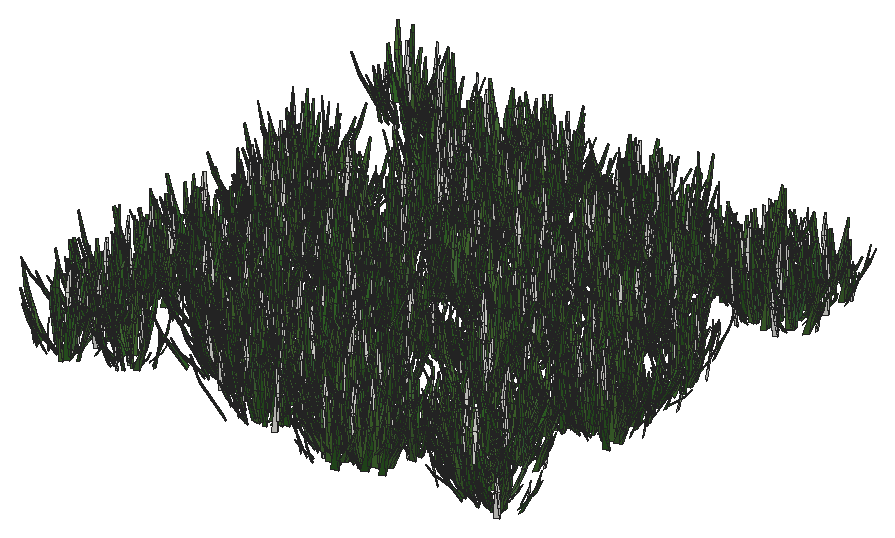
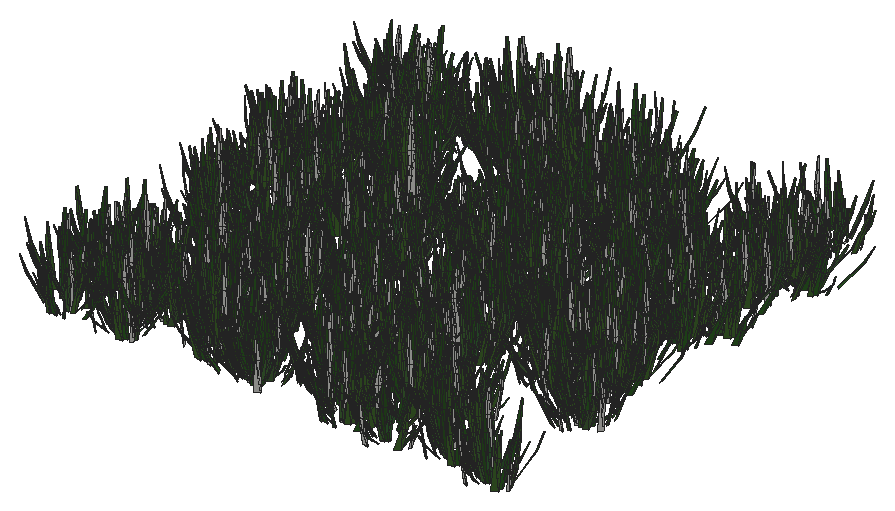
# SketchUp Ruby script. Lengths in inches.
U = 1.inch
M = Sketchup.active_model
def pt(a) = Geom::Point3d.new(a.map { |v| v * U })
def face(e, loops, mat)
  f = e.add_face(loops[0].map { |a| pt(a) })
  loops[1..].each { |l| e.add_face(l.map { |a| pt(a) }).erase! }
  f.material = f.back_material = mat if mat
  f
end
# faces: each face lists its corners as indices into pts; further lists are holes
def faces(e, pts, list, mat = nil) = list.each { |f| face(e, (f[0].is_a?(Array) ? f : [f]).map { |l| l.map { |i| pts[i] } }, mat) }
# xy, xz, yz: faces in a plane at the given z, y or x. An outline is a flat list of corners, or four numbers for a rectangle; further outlines are holes
def ring(l) = l.size == 4 ? [[l[0], l[1]], [l[2], l[1]], [l[2], l[3]], [l[0], l[3]]] : l.each_slice(2).to_a
def flat(e, list, mat, &to3) = list.each { |f| face(e, (f[0].is_a?(Array) ? f : [f]).map { |l| ring(l).map { |u, v| to3.(u, v) } }, mat) }
def xy(e, z, list, mat = nil) = flat(e, list, mat) { |x, y| [x, y, z] }
def xz(e, y, list, mat = nil) = flat(e, list, mat) { |x, z| [x, y, z] }
def yz(e, x, list, mat = nil) = flat(e, list, mat) { |y, z| [x, y, z] }
def lines(e, pts, list) = list.each { |a, b| e.add_line(pt(pts[a]), pt(pts[b])) }
# prism: a flat outline (further loops are holes) pulled along v
def prism(e, loops, v, mat = nil)
  f = face(e, loops, mat); d = Geom::Vector3d.new(v.map { |x| x * U })
  f.pushpull(f.normal.samedirection?(d) ? d.length : -d.length)
end
def box(e, o, s, mat = nil) = prism(e, [[o, [o[0] + s[0], o[1], o[2]], [o[0] + s[0], o[1] + s[1], o[2]], [o[0], o[1] + s[1], o[2]]]], [0, 0, s[2]], mat)
def at(x, y, z, deg = 0) = Geom::Transformation.translation(pt([x, y, z])) * Geom::Transformation.rotation(ORIGIN, Z_AXIS, deg.degrees)
def axes(o, x, y, z) = Geom::Transformation.new([*x, 0, *y, 0, *z, 0, *pt(o).to_a, 1])
def part(name) = M.definitions.add(name)
# library, detail: a bought-in or finely detailed component or shape, given as its bounding box
def library(name, o, s) = part(name).tap { |d| box(d.entities, o, s) }
def detail(e, o, s) = box(e.add_group.entities, o, s)
def put(e, d, t, mat = nil) = e.add_instance(d, t).tap { |i| i.material = mat if mat }
def group(e, t, mat = nil) = e.add_group.tap { |g| g.transformation = t; g.material = mat if mat }.entities
root = M.entities
M.materials.add("Material1").color = [58, 110, 58]
M.materials.add("Material10").color = [48, 100, 38]
M.materials.add("Material3").color = [68, 110, 58]
M.materials.add("Material4").color = [48, 90, 38]
M.materials.add("Material5").color = [68, 110, 48]
M.materials.add("Material6").color = [48, 90, 48]
M.materials.add("Material8").color = [58, 90, 38]
M.materials.add("Material9").color = [68, 100, 58]
c1 = part("grass00")
p = [[-0.6875,0.15,0],[-0.56,0.08,5.52],[-0.04,0.03,2.76],[0.48,-0.02,0],[0.35,-0.02,5.52],[-0.1,-0.14,5.52],
  [-0.12,0.65,8.37],[-0.42,0.65,8.37]]
faces(c1.entities,p,[[0,1,2,3],[3,2,4],[1,5,2],[5,4,2],[1,6,5],[4,5,6],[7,6,1]])
c2 = part("Group16\#1")
put(c2.entities,c1,axes([1.44,-0.61,-0.01],[0.05352,0.12609,0],[-0.10704,0.04543,0.07239],[0.06664,-0.02828,0.11628]),"Material6")
put(c2.entities,c1,axes([0.76,-0.15,-0.01],[0.04676,0.24062,0],[-0.23162,0.04501,0.06642],[0.0652,-0.01267,0.23595]),"Material3")
put(c2.entities,c1,axes([0.79,0.01,-0.01],[-0.00606,0.34651,0],[-0.34381,-0.00602,0.0432],[0.04319,0.00076,0.34386]))
put(c2.entities,c1,axes([1,0.23,-0.01],[-0.07192,0.31144,0],[-0.28722,-0.06632,0.1236],[0.12043,0.02781,0.29478]),"Material5")
put(c2.entities,c1,axes([1.66,0.77,-0.01],[-0.13828,0.29651,0],[-0.21551,-0.1005,0.22471],[0.20365,0.09498,0.23779]),"Material10")
put(c2.entities,c1,axes([0.6875,0.52,-0.01],[-0.18126,0.24051,0],[-0.22746,-0.17142,0.09788],[0.07817,0.05891,0.28481]),"Material5")
put(c2.entities,c1,axes([0.68,0.78,-0.01],[-0.215,0.18688,0],[-0.12385,-0.14248,0.21334],[0.13995,0.16101,0.18878]),"Material3")
put(c2.entities,c1,axes([0.56,1,-0.01],[-0.13756,0.07624,0],[-0.06159,-0.11112,0.0927],[0.04494,0.08108,0.12705]),"Material5")
put(c2.entities,c1,axes([0.2,0.64,-0.01],[-0.23729,0.07254,0],[-0.05711,-0.18681,0.153],[0.04473,0.14632,0.19535]),"Material10")
put(c2.entities,c1,axes([0.0625,0.72,-0.01],[-0.28874,0.02525,0],[-0.02179,-0.24916,0.14647],[0.01276,0.14591,0.25012]),"Material3")
put(c2.entities,c1,axes([-0.08,0.62,-0.01],[-0.34089,-0.04187,0],[0.03255,-0.26504,0.216],[-0.02633,0.21439,0.26703]),"Material10")
put(c2.entities,c1,axes([-0.34,0.98,-0.01],[-0.14314,-0.0493,0],[0.04397,-0.12769,0.06843],[-0.02228,0.0647,0.13505]),"Material10")
put(c2.entities,c1,axes([-0.87,1.45,-0.01],[-0.23488,-0.14114,0],[0.13761,-0.22901,0.06087],[-0.03135,0.05217,0.26717]))
put(c2.entities,c1,axes([-0.72,0.77,-0.01],[-0.14208,-0.13251,0],[0.07209,-0.0773,0.16301],[-0.11118,0.11922,0.1057]),"Material10")
put(c2.entities,c1,axes([-0.62,0.43,-0.01],[-0.14845,-0.21203,0],[0.18654,-0.13061,0.12304],[-0.10079,0.07057,0.22772]),"Material3")
put(c2.entities,c1,axes([-0.68,0.29,-0.01],[-0.13639,-0.32136,0],[0.31723,-0.13464,0.05579],[-0.05136,0.0218,0.34462]),"Material4")
put(c2.entities,c1,axes([-0.64,0.125,-0.01],[-0.0458,-0.23569,0],[0.22124,-0.043,0.08276],[-0.08124,0.01579,0.22538]),"Material1")
put(c2.entities,c1,axes([-1.6,-0.03,-0.01],[0.00576,-0.32897,0],[0.27526,0.00482,0.18018],[-0.18015,-0.00315,0.2753]),"Material5")
put(c2.entities,c1,axes([-1.36,-0.31,-0.01],[0.05718,-0.24765,0],[0.18172,0.04196,0.17267],[-0.16825,-0.03885,0.1865]),"Material10")
put(c2.entities,c1,axes([-1.54,-0.72,-0.01],[0.06537,-0.14017,0],[0.13555,0.06321,0.03939],[-0.0357,-0.01665,0.14956]))
put(c2.entities,c1,axes([-1.19,-0.9,-0.01],[0.09597,-0.12735,0],[0.11214,0.08451,0.07557],[-0.06035,-0.04548,0.14042]),"Material9")
put(c2.entities,c1,axes([-0.47,-0.54,-0.01],[0.11588,-0.10072,0],[0.0618,0.0711,0.12124],[-0.07953,-0.0915,0.0942]))
put(c2.entities,c1,axes([-0.47,-0.84,-0.01],[0.11927,-0.0661,0],[0.06603,0.11913,0.00646],[-0.00313,-0.00565,0.13621]),"Material5")
put(c2.entities,c1,axes([-0.38,-1.24,-0.01],[0.28037,-0.08571,0],[0.0618,0.20215,0.20315],[-0.05939,-0.19428,0.21139]),"Material9")
put(c2.entities,c1,axes([-0.06,-0.66,-0.01],[0.22719,-0.01987,0],[0.01247,0.14255,0.17758],[-0.01547,-0.17691,0.1431]),"Material8")
put(c2.entities,c1,axes([0.11,-0.89,-0.01],[0.14882,0.01828,0],[-0.01058,0.08611,0.12229],[0.01491,-0.12138,0.08676]),"Material6")
put(c2.entities,c1,axes([0.25,-0.72,-0.01],[0.20481,0.07053,0],[-0.06206,0.18022,0.10291],[0.03351,-0.0973,0.1906]),"Material6")
put(c2.entities,c1,axes([0.85,-1.42,-0.01],[0.16481,0.09904,0],[-0.09472,0.15762,0.05616],[0.02893,-0.04814,0.18389]),"Material5")
put(c2.entities,c1,axes([1.01,-1.09,-0.01],[0.21858,0.20385,0],[-0.17495,0.1876,0.15339],[0.10462,-0.11218,0.25652]),"Material10")
put(c2.entities,c1,axes([1.01,-0.71,-0.01],[0.08733,0.12473,0],[-0.06445,0.04512,0.13037],[0.1068,-0.07477,0.07867]),"Material6")
c3 = part("Group15\#1")
put(c3.entities,c2,at(0,0,0))
c4 = part("3darcstudiotree_grass00\#1")
put(c4.entities,c3,at(0,0,0))
put(root,c4,axes([268.16,97.04,0.25],[1.10424,-0.06793,0],[0.07798,0.87325,-0.02045],[0.00258,0.02892,1.8024]))
put(root,c4,axes([287.49,97.18,0.25],[0.30872,-0.99726,0],[1.14542,0.24428,-0.01129],[0.01726,0.00368,1.86628]))
put(root,c4,axes([288.79,97.94,0.25],[0.3848,-0.95006,0],[1.16691,0.32559,-0.02131],[0.02787,0.00778,1.69918]))
put(root,c4,axes([289.95,98.12,0.25],[0.36065,-0.88025,0],[1.08014,0.30487,-0.01889],[0.03083,0.0087,1.96679]))
put(root,c4,axes([281.65,97.91,0.25],[-1.09019,-0.50143,0],[0.60004,-0.89873,-0.02403],[0.01807,-0.02706,1.92026]))
put(root,c4,axes([271.9375,98.29,0.25],[0.34802,0.74456,0],[-0.96206,0.30978,-0.02781],[-0.03955,0.01273,1.57422]))
put(root,c4,axes([298.37,98.26,0.25],[-1.11705,-0.08782,0],[0.09396,-0.82334,-0.02721],[0.00339,-0.02975,1.31849]))
put(root,c4,axes([286.48,98.61,0.25],[0.24214,0.73963,0],[-0.93506,0.21089,-0.02204],[-0.04106,0.00926,1.87051]))
put(root,c4,axes([282.78,99.14,0.25],[1.15932,-0.25477,0],[0.28267,0.88609,-0.03329],[0.01046,0.0328,1.35616]))
put(root,c4,axes([296.02,99.06,0.25],[-0.27861,0.84951,0],[-1.24912,-0.28222,-0.0223],[-0.02643,-0.00597,1.58974]))
put(root,c4,axes([280,99.92,0.25],[0.8678,0.26913,0],[-0.39255,0.87201,-0.02415],[-0.01451,0.03224,1.92547]))
put(root,c4,axes([269.21,99.85,0.25],[-0.87323,0.18273,0],[-0.30243,-0.99566,-0.01943],[-0.00513,-0.01691,1.33771]))
put(root,c4,axes([295.06,100.45,0.25],[0.23734,-0.94344,0],[1.1996,0.20789,-0.01659],[0.02057,0.00357,1.55232]))
put(root,c4,axes([290.86,100.39,0.25],[0.77506,0.65428,0],[-0.89383,0.72943,-0.00938],[-0.01044,0.00852,1.95578]))
put(root,c4,axes([288.87,100.38,0.25],[0.63502,0.71653,0],[-0.97082,0.59271,-0.02079],[-0.01883,0.0115,1.35493]))
put(root,c4,axes([278.34,100.35,0.25],[-1.08362,-0.14985,0],[0.15604,-0.77736,-0.01531],[0.00477,-0.02379,1.80136]))
put(root,c4,axes([277.1,100.4,0.25],[-1.24003,0.01344,0],[-0.01576,-1.00201,-0.02897],[-0.00045,-0.02857,1.4344]))
put(root,c4,axes([267.86,100.45,0.25],[-1.00644,0.0521,0],[-0.07788,-1.03631,-0.0193],[-0.00128,-0.01707,1.33558]))
put(root,c4,axes([283.02,101.13,0.25],[-0.82708,0.70088,0],[-0.92501,-0.75198,-0.0181],[-0.01933,-0.01572,1.93624]))
put(root,c4,axes([267.73,101.61,0.25],[-0.68746,0.64244,0],[-0.83442,-0.61511,-0.01682],[-0.01762,-0.01299,1.56312]))
put(root,c4,axes([266.57,101.82,0.25],[-1.25746,-0.26238,0],[0.23041,-0.76071,-0.02201],[0.00764,-0.02522,1.34565]))
put(root,c4,axes([276.43,102.16,0.25],[0.01562,-0.76739,0],[1.27864,0.01793,-0.02351],[0.02966,0.00042,1.61343]))
put(root,c4,axes([278.43,102.34,0.25],[0.80377,-0.68068,0],[0.75481,0.61403,-0.0131],[0.01592,0.01295,1.79861]))
put(root,c4,axes([293,101.99,0.25],[-0.26779,0.87549,0],[-1.041,-0.21936,-0.01715],[-0.02259,-0.00476,1.46021]))
put(root,c4,axes([285.55,102.18,0.25],[-0.96262,0.33739,0],[-0.48324,-0.94982,-0.01449],[-0.00747,-0.01469,1.64714]))
put(root,c4,axes([295.38,102.4,0.25],[0.73171,0.79313,0],[-0.89991,0.57195,-0.02004],[-0.01916,0.01218,1.3651]))
put(root,c4,axes([278.3,102.81,0.25],[0.25731,-0.93118,0],[0.9412,0.17917,-0.013],[0.02579,0.00491,1.96601]))
put(root,c4,axes([275.79,103.09,0.25],[-0.84078,-0.75319,0],[0.89143,-0.68552,-0.02123],[0.01845,-0.01419,1.43939]))
put(root,c4,axes([284.42,103.4375,0.25],[0.78957,-0.53115,0],[0.75361,0.77175,-0.02341],[0.01959,0.02007,1.59067]))
put(root,c4,axes([276.82,103.24,0.25],[-0.86189,-0.77183,0],[0.84517,-0.65017,-0.01903],[0.02326,-0.01789,1.91973]))
put(root,c4,axes([296.06,103.1,0.25],[-1.12646,0.29609,0],[-0.30982,-0.81199,-0.01419],[-0.00731,-0.01915,1.75006]))
put(root,c4,axes([280.9375,103.14,0.25],[-1.01462,0.45633,0],[-0.60435,-0.92569,-0.0133],[-0.00973,-0.0149,1.94738]))
put(root,c4,axes([267.68,103.67,0.25],[1.23208,0.08593,0],[-0.08825,0.87173,-0.00911],[-0.00141,0.01392,1.94776]))
put(root,c4,axes([285.47,103.625,0.25],[-1.14143,-0.12101,0],[0.13671,-0.88832,-0.0157],[0.00356,-0.02311,1.92971]))
put(root,c4,axes([272.01,104.4,0.25],[0.93086,0.02644,0],[-0.04238,1.028,-0.02332],[-0.00116,0.02823,1.80921]))
put(root,c4,axes([273.86,104.35,0.25],[-0.25152,-0.74059,0],[1.23081,-0.28797,-0.01485],[0.02017,-0.00472,1.80381]))
put(root,c4,axes([274.79,105.72,0.25],[0.27103,-0.82455,0],[1.10427,0.25005,-0.01691],[0.02285,0.00517,1.6028]))
put(root,c4,axes([268.22,105.35,0.25],[-0.89891,0.66342,0],[-0.73857,-0.68941,-0.01814],[-0.01883,-0.01757,1.73642]))
put(root,c4,axes([293.78,105.83,0.25],[0.11242,-0.76343,0],[1.17967,0.11967,-0.02785],[0.03483,0.00353,1.49696]))
put(root,c4,axes([280.3,105.87,0.25],[0.91228,0.21916,0],[-0.30497,0.87453,-0.02015],[-0.00837,0.02399,1.63787]))
put(root,c4,axes([284.75,105.78,0.25],[-0.8369,-0.47794,0],[0.58779,-0.70905,-0.02104],[0.01995,-0.02407,1.73448]))
put(root,c4,axes([290.6,106.1,0.25],[0.98705,-0.26516,0],[0.36613,0.93893,-0.01611],[0.0066,0.01692,1.58139]))
put(root,c4,axes([272.8125,106.18,0.25],[1.25165,0.05796,0],[-0.05382,0.80063,-0.03032],[-0.00269,0.04005,1.54015]))
put(root,c4,axes([276.66,105.91,0.25],[-0.47261,0.91291,0],[-0.90808,-0.32386,-0.02574],[-0.03173,-0.01132,1.32606]))
put(root,c4,axes([281.34,106.98,0.25],[1.10757,0.16543,0],[-0.2285,1.05392,-0.01866],[-0.0044,0.02028,1.717]))
put(root,c4,axes([294.84,106.73,0.25],[0.38124,0.81676,0],[-0.87245,0.28054,-0.02409],[-0.03859,0.01241,1.60735]))
put(root,c4,axes([274.01,107.16,0.25],[0.72633,-0.56205,0],[0.87867,0.78223,-0.02398],[0.01751,0.01559,1.37951]))
put(root,c4,axes([275.34,107.1875,0.25],[-0.88877,0.23914,0],[-0.31177,-0.79822,-0.02033],[-0.01193,-0.03054,1.92362]))
put(root,c4,axes([290.09,107.86,0.25],[-0.85116,0.74725,0],[-0.72534,-0.56917,-0.02847],[-0.02911,-0.02284,1.40417]))
put(root,c4,axes([295.29,108.6,0.25],[1.01087,-0.15503,0],[0.22739,1.02141,-0.01263],[0.00318,0.01427,1.73191]))
put(root,c4,axes([296.85,108.44,0.25],[-0.7743,-0.53232,0],[0.66052,-0.66187,-0.01497],[0.01682,-0.01686,1.82381]))
put(root,c4,axes([298.45,108.72,0.25],[0.07297,-0.99898,0],[1.1057,0.05564,-0.02606],[0.03951,0.00199,1.68211]))
put(root,c4,axes([266.57,108.62,0.25],[-0.50796,0.79425,0],[-0.91074,-0.40126,-0.02935],[-0.03326,-0.01466,1.32321]))
put(root,c4,axes([297.81,109.53,0.25],[0.00661,-0.76532,0],[0.95296,0.00567,-0.01704],[0.03212,0.00019,1.79616]))
put(root,c4,axes([288.67,109.75,0.25],[0.51631,-0.92665,0],[1.17058,0.44932,-0.01],[0.01399,0.00537,1.98774]))
put(root,c4,axes([278.17,109.54,0.25],[0.98417,0.64292,0],[-0.72581,0.7654,-0.01986],[-0.02023,0.02134,1.93312]))
put(root,c4,axes([283.22,109.81,0.25],[0.31191,-0.76511,0],[1.09515,0.30756,-0.02846],[0.0314,0.00882,1.34635]))
put(root,c4,axes([272.54,109.67,0.25],[-1.25339,0.20143,0],[-0.24239,-1.03905,-0.01839],[-0.00413,-0.01772,1.50803]))
put(root,c4,axes([285.46,109.99,0.25],[-0.4345,-0.70478,0],[1.06416,-0.45196,-0.02541],[0.025,-0.01062,1.32108]))
put(root,c4,axes([268.26,109.83,0.25],[-0.75518,0.67832,0],[-0.91766,-0.70381,-0.01856],[-0.02014,-0.01545,1.84646]))
put(root,c4,axes([295.21,110.44,0.25],[0.92845,-0.66262,0],[0.58735,0.56696,-0.0226],[0.02712,0.02618,1.65792]))
put(root,c4,axes([281.12,110.63,0.25],[-0.9762,-0.51258,0],[0.63746,-0.83634,-0.01513],[0.0122,-0.01601,1.79885]))
put(root,c4,axes([279.33,110.92,0.25],[-0.80163,-0.4961,0],[0.69067,-0.76883,-0.01853],[0.01459,-0.01624,1.52144]))
put(root,c4,axes([268.29,110.99,0.25],[-1.10301,-0.18835,0],[0.23802,-0.96027,-0.02294],[0.00674,-0.02721,1.72347]))
put(root,c4,axes([297.82,111.125,0.25],[-0.65227,0.61485,0],[-0.88094,-0.64381,-0.02335],[-0.02496,-0.01824,1.67208]))
put(root,c4,axes([271.8,111.28,0.25],[-0.26759,1.02243,0],[-1.03741,-0.18705,-0.03052],[-0.03905,-0.00704,1.38983]))
put(root,c4,axes([270.74,111.85,0.25],[-0.93432,-0.19513,0],[0.23337,-0.7698,-0.02412],[0.00996,-0.03286,1.61843]))
put(root,c4,axes([289.39,112.25,0.25],[-0.16519,0.86896,0],[-1.05038,-0.13756,-0.0149],[-0.02658,-0.00348,1.9212]))
put(root,c4,axes([276.53,112.32,0.25],[-1.24011,-0.05471,0],[0.06269,-0.97897,-0.02618],[0.00204,-0.03185,1.73378]))
put(root,c4,axes([275.16,112.48,0.25],[-0.59447,0.58786,0],[-0.79237,-0.552,-0.02769],[-0.03072,-0.0214,1.49833]))
put(root,c4,axes([297.91,112.89,0.25],[-0.34351,-0.85877,0],[1.01547,-0.27983,-0.03393],[0.03976,-0.01096,1.3212]))
put(root,c4,axes([270.81,113.13,0.25],[0.93424,-0.68706,0],[0.77952,0.73022,-0.01442],[0.01553,0.01455,1.90876]))
put(root,c4,axes([287.3125,113.4375,0.25],[1.10079,-0.06818,0],[0.07524,0.83691,-0.02534],[0.00295,0.03282,1.58232]))
put(root,c4,axes([292.4,113.21,0.25],[0.48218,0.91637,0],[-0.93085,0.33742,-0.01938],[-0.02779,0.01007,1.58937]))
put(root,c4,axes([269.16,113.15,0.25],[-0.8368,0.51903,0],[-0.54055,-0.60038,-0.01872],[-0.02016,-0.02239,1.62421]))
put(root,c4,axes([286.1,113.73,0.25],[0.69341,-0.64478,0],[0.94398,0.69935,-0.02458],[0.0259,0.01919,1.78746]))
put(root,c4,axes([276.36,113.66,0.25],[0.03328,-0.93429,0],[1.20344,0.02953,-0.0158],[0.02262,0.00056,1.72451]))
put(root,c4,axes([280.38,113.59,0.25],[-0.28609,-0.73195,0],[1.12202,-0.30212,-0.01227],[0.01821,-0.0049,1.83962]))
put(root,c4,axes([288.41,113.79,0.25],[0.87385,-0.65283,0],[0.6668,0.61487,-0.02235],[0.02902,0.02676,1.93391]))
put(root,c4,axes([277.93,114.49,0.25],[1.0866,-0.33924,0],[0.36466,0.80465,-0.01237],[0.00777,0.01715,1.84855]))
put(root,c4,axes([269.61,114.6,0.25],[0.2213,-0.80151,0],[1.05711,0.20107,-0.01662],[0.02709,0.00515,1.81323]))
put(root,c4,axes([271.83,114.35,0.25],[-0.96141,-0.08719,0],[0.13518,-1.0268,-0.01667],[0.00261,-0.01979,1.79039]))
put(root,c4,axes([284.71,114.77,0.25],[1.02851,0.16815,0],[-0.23702,0.99873,-0.03192],[-0.00732,0.03084,1.45488]))
put(root,c4,axes([271.24,114.81,0.25],[0.91803,-0.28549,0],[0.33346,0.7387,-0.02122],[0.01473,0.03264,1.88089]))
put(root,c4,axes([277.18,114.92,0.25],[0.6036,-0.90128,0],[0.84793,0.39121,-0.02727],[0.03552,0.01639,1.44583]))
put(root,c4,axes([289.33,114.85,0.25],[-0.74245,0.5983,0],[-0.81625,-0.69779,-0.01854],[-0.01963,-0.01678,1.78092]))
put(root,c4,axes([281.55,115.4,0.25],[0.93643,0.55966,0],[-0.58159,0.67039,-0.02682],[-0.02773,0.03197,1.76121]))
put(root,c4,axes([269.54,115.82,0.25],[-0.24487,-0.96185,0],[1.15857,-0.20319,-0.02196],[0.03265,-0.00573,1.79942]))
put(root,c4,axes([273.71,115.67,0.25],[-0.88791,-0.35527,0],[0.40268,-0.6933,-0.00927],[0.00865,-0.0149,1.99366]))
put(root,c4,axes([297.61,116.01,0.25],[0.26325,-0.80283,0],[0.90673,0.20482,-0.01758],[0.03099,0.007,1.71636]))
put(root,c4,axes([267.54,115.77,0.25],[-0.98413,0.25809,0],[-0.31982,-0.8401,-0.02199],[-0.00939,-0.02468,1.50537]))
put(root,c4,axes([293.43,116.95,0.25],[-0.1853,-0.97395,0],[1.14146,-0.14961,-0.01303],[0.02193,-0.00287,1.96953]))
put(root,c4,axes([292.14,116.69,0.25],[-0.82467,0.67334,0],[-0.67813,-0.57216,-0.0233],[-0.03099,-0.02615,1.83382]))
put(root,c4,axes([270.71,116.7,0.25],[-0.9032,0.46383,0],[-0.60843,-0.81618,-0.03047],[-0.01925,-0.02582,1.38852]))
put(root,c4,axes([268.01,117.32,0.25],[-0.85157,0.62189,0],[-0.70382,-0.66393,-0.02195],[-0.02479,-0.02338,1.82186]))
put(root,c4,axes([267.76,118.04,0.25],[0.43488,-0.96189,0],[0.88058,0.27426,-0.02337],[0.03887,0.01211,1.67088]))
put(root,c4,axes([271.03,118.01,0.25],[-0.08379,-0.93247,0],[1.23367,-0.07636,-0.02024],[0.03008,-0.00186,1.84439]))
put(root,c4,axes([285.5,118.25,0.25],[1.08793,-0.00248,0],[0.00317,0.9599,-0.02008],[0.00008,0.02329,1.61638]))
put(root,c4,axes([275.39,118.38,0.25],[1.08731,-0.07688,0],[0.08315,0.81014,-0.01096],[0.00184,0.01791,1.93666]))
put(root,c4,axes([279.87,118.32,0.25],[0.34854,0.94579,0],[-1.21535,0.30855,-0.03143],[-0.03382,0.00859,1.42994]))
put(root,c4,axes([296.11,118.47,0.25],[-0.96913,-0.31436,0],[0.36973,-0.78522,-0.02269],[0.01336,-0.02837,1.64292]))
put(root,c4,axes([292.07,118.42,0.25],[-0.19535,0.90119,0],[-1.13567,-0.16959,-0.02584],[-0.02869,-0.00428,1.30174]))
put(root,c4,axes([287.06,118.56,0.25],[0.25187,0.74896,0],[-0.89201,0.20665,-0.02635],[-0.03964,0.00918,1.4463]))
put(root,c4,axes([276.38,119.86,0.25],[0.91828,-0.36415,0],[0.4413,0.76663,-0.01719],[0.01234,0.02143,1.70421]))
put(root,c4,axes([282.72,119.89,0.25],[0.50712,-0.65796,0],[0.93935,0.49876,-0.02581],[0.03144,0.01669,1.61243]))
put(root,c4,axes([270.64,119.54,0.25],[-0.43653,0.75716,0],[-1.07031,-0.4251,-0.03408],[-0.03517,-0.01397,1.35762]))
put(root,c4,axes([292.55,120.51,0.25],[0.96053,-0.32125,0],[0.34403,0.70863,-0.02314],[0.01263,0.02602,1.34449]))
put(root,c4,axes([275.6,120.72,0.25],[1.19135,-0.36369,0],[0.38992,0.87991,-0.01984],[0.01158,0.02612,1.90869]))
put(root,c4,axes([279.32,120.78,0.25],[-1.13557,0.0762,0],[-0.07638,-0.78423,-0.02584],[-0.00383,-0.03931,1.74304]))
put(root,c4,axes([289.47,121.01,0.25],[-1.20827,-0.38463,0],[0.44631,-0.96583,-0.02874],[0.01106,-0.02393,1.33872]))
put(root,c4,axes([266.36,121.23,0.25],[0.89225,0.40196,0],[-0.55877,0.85447,-0.01651],[-0.01218,0.01862,1.81134]))
put(root,c4,axes([292.39,121.86,0.25],[0.54452,-0.65159,0],[1.06707,0.61431,-0.02169],[0.0216,0.01244,1.57389]))
put(root,c4,axes([266.64,121.83,0.25],[-0.40062,-0.97292,0],[1.04571,-0.29663,-0.03013],[0.03964,-0.01125,1.53631]))
put(root,c4,axes([286,122.07,0.25],[0.64009,-0.73264,0],[0.94558,0.56913,-0.00976],[0.01281,0.00771,1.89325]))
put(root,c4,axes([281.54,121.85,0.25],[-0.73071,0.76198,0],[-0.82282,-0.54358,-0.02078],[-0.02855,-0.01886,1.84714]))
put(root,c4,axes([286.96,122.17,0.25],[-0.87163,0.5354,0],[-0.68211,-0.765,-0.01624],[-0.01535,-0.01721,1.82169]))
put(root,c4,axes([278.7,122.43,0.25],[0.47221,0.99651,0],[-1.08054,0.35274,-0.01805],[-0.02754,0.00899,1.90362]))
put(root,c4,axes([280.26,123.45,0.25],[0.38437,-0.76536,0],[1.0026,0.34687,-0.02113],[0.02721,0.00941,1.51549]))
put(root,c4,axes([290.21,123.16,0.25],[-0.94119,0.32809,0],[-0.39966,-0.78983,-0.01995],[-0.01215,-0.024,1.62326]))
put(root,c4,axes([287.19,123.82,0.25],[-0.49188,-0.70517,0],[0.9641,-0.46328,-0.02105],[0.03177,-0.01527,1.94345]))
put(root,c4,axes([274.05,124.24,0.25],[0.8215,-0.69363,0],[0.71096,0.58007,-0.02297],[0.02754,0.02247,1.67632]))
put(root,c4,axes([296.4,124.29,0.25],[-0.82065,0.53258,0],[-0.63041,-0.66919,-0.02144],[-0.02509,-0.02663,1.94421]))
put(root,c4,axes([281.41,124.5,0.25],[-1.10863,0.03131,0],[-0.04139,-1.0095,-0.01213],[-0.00063,-0.01543,1.86653]))
put(root,c4,axes([276.9,124.85,0.25],[-0.32692,-0.77468,0],[0.87231,-0.2536,-0.02961],[0.04062,-0.01181,1.34337]))
put(root,c4,axes([287.18,124.57,0.25],[-0.5593,0.85438,0],[-1.02617,-0.46278,-0.0267],[-0.02647,-0.01194,1.31753]))
put(root,c4,axes([289.94,125.01,0.25],[0.99343,0.20197,0],[-0.30646,1.03848,-0.01455],[-0.00532,0.01802,1.97892]))
put(root,c4,axes([271.94,125.04,0.25],[0.40737,0.76752,0],[-0.96023,0.3511,-0.02705],[-0.03635,0.01329,1.54111]))
put(root,c4,axes([298.36,124.95,0.25],[-0.98153,0.27111,0],[-0.38749,-0.96645,-0.02244],[-0.00941,-0.02347,1.62972]))
put(root,c4,axes([291.59,125.03,0.25],[-0.97723,0.56468,0],[-0.69575,-0.82947,-0.02528],[-0.02097,-0.025,1.76765]))
put(root,c4,axes([292.52,125.7,0.25],[0.46054,-0.84804,0],[0.8307,0.31078,-0.02223],[0.03624,0.01356,1.62899]))
put(root,c4,axes([294.84,125.77,0.25],[0.09125,-0.97276,0],[1.05287,0.06804,-0.01871],[0.0317,0.00205,1.79426]))
put(root,c4,axes([296.85,125.86,0.25],[0.86878,-0.2882,0],[0.45635,0.94771,-0.02256],[0.01062,0.02205,1.55958]))
put(root,c4,axes([275.17,125.5,0.25],[-0.94522,0.15916,0],[-0.19762,-0.80852,-0.01756],[-0.00621,-0.02539,1.76676]))
put(root,c4,axes([278.24,125.61,0.25],[-1.2125,-0.19056,0],[0.20846,-0.91376,-0.02653],[0.00747,-0.03272,1.69452]))
put(root,c4,axes([279.48,127.08,0.25],[0.10531,-0.99553,0],[1.0274,0.07487,-0.02351],[0.03748,0.00273,1.65028]))
put(root,c4,axes([272.41,126.76,0.25],[-0.95102,0.27714,0],[-0.33621,-0.7948,-0.01418],[-0.0084,-0.01986,1.8149]))
put(root,c4,axes([292.32,127.06,0.25],[-0.54208,-0.96431,0],[1.05962,-0.41035,-0.01753],[0.02036,-0.00788,1.49864]))
put(root,c4,axes([293.99,126.87,0.25],[0.22308,1.02176,0],[-1.21601,0.18289,-0.02342],[-0.03183,0.00479,1.70718]))
put(root,c4,axes([274.77,127.22,0.25],[-0.62075,0.54549,0],[-0.89288,-0.69998,-0.01576],[-0.0175,-0.01372,1.87507]))
put(root,c4,axes([278.8,128.125,0.25],[1.1647,-0.31861,0],[0.33612,0.84645,-0.0158],[0.00908,0.02288,1.97161]))
put(root,c4,axes([279.86,127.97,0.25],[-1.15241,0.07959,0],[-0.08162,-0.81413,-0.01346],[-0.00195,-0.01947,1.72106]))
put(root,c4,axes([297.82,128.15,0.25],[-1.06269,-0.32453,0],[0.42482,-0.95833,-0.01333],[0.00645,-0.01455,1.7245]))
put(root,c4,axes([283.92,128.64,0.25],[-0.37342,-0.88106,0],[0.93238,-0.27224,-0.03242],[0.0414,-0.01209,1.33794]))
put(root,c4,axes([287.47,128.73,0.25],[-0.17239,-0.74153,0],[1.2439,-0.19921,-0.02161],[0.03277,-0.00525,1.95654]))
put(root,c4,axes([285.38,128.55,0.25],[-0.97399,-0.21425,0],[0.25281,-0.79174,-0.01321],[0.00667,-0.02089,1.9444]))
put(root,c4,axes([284.02,129.32,0.25],[1.18946,0.11559,0],[-0.14498,1.02777,-0.02723],[-0.00408,0.02894,1.60719]))
put(root,c4,axes([269.55,129.41,0.25],[0.46251,-0.74808,0],[1.00872,0.42963,-0.0206],[0.02836,0.01208,1.75423]))
put(root,c4,axes([293.18,129.84,0.25],[0.36361,-0.70141,0],[1.00069,0.35737,-0.02985],[0.03887,0.01388,1.54439]))
put(root,c4,axes([274.03,130.01,0.25],[1.04396,-0.63723,0],[0.70689,0.79781,-0.02397],[0.01576,0.01779,1.32443]))
put(root,c4,axes([297.63,129.68,0.25],[-0.94731,0.6131,0],[-0.56659,-0.6031,-0.02241],[-0.02209,-0.02351,1.47722]))
put(root,c4,axes([266.36,130.16,0.25],[0.77656,-0.71212,0],[0.86276,0.64814,-0.01132],[0.0132,0.00992,1.83032]))
put(root,c4,axes([277.18,129.83,0.25],[-0.6204,0.76817,0],[-0.85337,-0.4748,-0.02214],[-0.02926,-0.01628,1.63462]))
